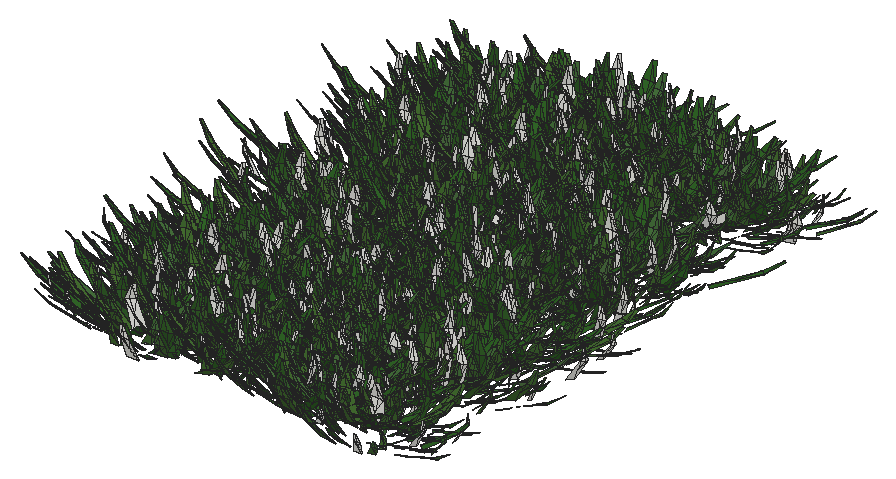
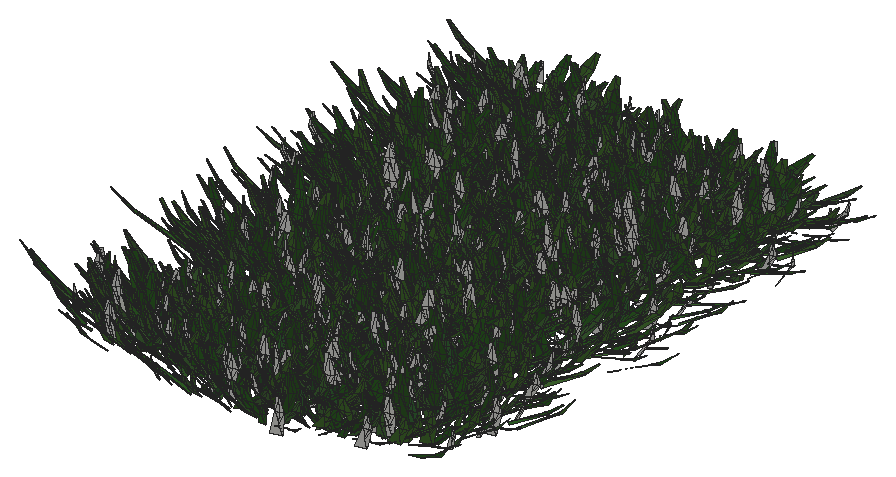
# SketchUp Ruby script. Lengths in inches.
U = 1.inch
M = Sketchup.active_model
def pt(a) = Geom::Point3d.new(a.map { |v| v * U })
def face(e, loops, mat)
  f = e.add_face(loops[0].map { |a| pt(a) })
  loops[1..].each { |l| e.add_face(l.map { |a| pt(a) }).erase! }
  f.material = f.back_material = mat if mat
  f
end
# faces: each face lists its corners as indices into pts; further lists are holes
def faces(e, pts, list, mat = nil) = list.each { |f| face(e, (f[0].is_a?(Array) ? f : [f]).map { |l| l.map { |i| pts[i] } }, mat) }
# xy, xz, yz: faces in a plane at the given z, y or x. An outline is a flat list of corners, or four numbers for a rectangle; further outlines are holes
def ring(l) = l.size == 4 ? [[l[0], l[1]], [l[2], l[1]], [l[2], l[3]], [l[0], l[3]]] : l.each_slice(2).to_a
def flat(e, list, mat, &to3) = list.each { |f| face(e, (f[0].is_a?(Array) ? f : [f]).map { |l| ring(l).map { |u, v| to3.(u, v) } }, mat) }
def xy(e, z, list, mat = nil) = flat(e, list, mat) { |x, y| [x, y, z] }
def xz(e, y, list, mat = nil) = flat(e, list, mat) { |x, z| [x, y, z] }
def yz(e, x, list, mat = nil) = flat(e, list, mat) { |y, z| [x, y, z] }
def lines(e, pts, list) = list.each { |a, b| e.add_line(pt(pts[a]), pt(pts[b])) }
# prism: a flat outline (further loops are holes) pulled along v
def prism(e, loops, v, mat = nil)
  f = face(e, loops, mat); d = Geom::Vector3d.new(v.map { |x| x * U })
  f.pushpull(f.normal.samedirection?(d) ? d.length : -d.length)
end
def box(e, o, s, mat = nil) = prism(e, [[o, [o[0] + s[0], o[1], o[2]], [o[0] + s[0], o[1] + s[1], o[2]], [o[0], o[1] + s[1], o[2]]]], [0, 0, s[2]], mat)
def at(x, y, z, deg = 0) = Geom::Transformation.translation(pt([x, y, z])) * Geom::Transformation.rotation(ORIGIN, Z_AXIS, deg.degrees)
def axes(o, x, y, z) = Geom::Transformation.new([*x, 0, *y, 0, *z, 0, *pt(o).to_a, 1])
def part(name) = M.definitions.add(name)
# library, detail: a bought-in or finely detailed component or shape, given as its bounding box
def library(name, o, s) = part(name).tap { |d| box(d.entities, o, s) }
def detail(e, o, s) = box(e.add_group.entities, o, s)
def put(e, d, t, mat = nil) = e.add_instance(d, t).tap { |i| i.material = mat if mat }
def group(e, t, mat = nil) = e.add_group.tap { |g| g.transformation = t; g.material = mat if mat }.entities
root = M.entities
M.materials.add("Material82").color = [68, 110, 58]
M.materials.add("Material83").color = [48, 90, 38]
M.materials.add("Material84").color = [68, 110, 48]
M.materials.add("Material85").color = [48, 90, 48]
M.materials.add("Material86").color = [58, 110, 58]
M.materials.add("Material87").color = [58, 90, 38]
M.materials.add("Material88").color = [68, 100, 58]
M.materials.add("Material89").color = [48, 100, 38]
c1 = part("grass00")
p = [[-0.6875,0.15,0],[-0.56,0.08,5.52],[-0.04,0.03,2.76],[0.48,-0.02,0],[0.35,-0.02,5.52],[-0.1,-0.14,5.52],
  [-0.12,0.65,8.37],[-0.42,0.65,8.37]]
faces(c1.entities,p,[[0,1,2,3],[3,2,4],[1,5,2],[5,4,2],[1,6,5],[4,5,6],[7,6,1]])
c2 = part("Group16\#1")
put(c2.entities,c1,axes([1.44,-0.61,-0.01],[0.05352,0.12609,0],[-0.10704,0.04543,0.07239],[0.06664,-0.02828,0.11628]),"Material85")
put(c2.entities,c1,axes([0.76,-0.15,-0.01],[0.04676,0.24062,0],[-0.23162,0.04501,0.06642],[0.0652,-0.01267,0.23595]),"Material82")
put(c2.entities,c1,axes([0.79,0.01,-0.01],[-0.00606,0.34651,0],[-0.34381,-0.00602,0.0432],[0.04319,0.00076,0.34386]))
put(c2.entities,c1,axes([1,0.23,-0.01],[-0.07192,0.31144,0],[-0.28722,-0.06632,0.1236],[0.12043,0.02781,0.29478]),"Material84")
put(c2.entities,c1,axes([1.66,0.77,-0.01],[-0.13828,0.29651,0],[-0.21551,-0.1005,0.22471],[0.20365,0.09498,0.23779]),"Material89")
put(c2.entities,c1,axes([0.6875,0.52,-0.01],[-0.18126,0.24051,0],[-0.22746,-0.17142,0.09788],[0.07817,0.05891,0.28481]),"Material84")
put(c2.entities,c1,axes([0.68,0.78,-0.01],[-0.215,0.18688,0],[-0.12385,-0.14248,0.21334],[0.13995,0.16101,0.18878]),"Material82")
put(c2.entities,c1,axes([0.56,1,-0.01],[-0.13756,0.07624,0],[-0.06159,-0.11112,0.0927],[0.04494,0.08108,0.12705]),"Material84")
put(c2.entities,c1,axes([0.2,0.64,-0.01],[-0.23729,0.07254,0],[-0.05711,-0.18681,0.153],[0.04473,0.14632,0.19535]),"Material89")
put(c2.entities,c1,axes([0.0625,0.72,-0.01],[-0.28874,0.02525,0],[-0.02179,-0.24916,0.14647],[0.01276,0.14591,0.25012]),"Material82")
put(c2.entities,c1,axes([-0.08,0.62,-0.01],[-0.34089,-0.04187,0],[0.03255,-0.26504,0.216],[-0.02633,0.21439,0.26703]),"Material89")
put(c2.entities,c1,axes([-0.34,0.98,-0.01],[-0.14314,-0.0493,0],[0.04397,-0.12769,0.06843],[-0.02228,0.0647,0.13505]),"Material89")
put(c2.entities,c1,axes([-0.87,1.45,-0.01],[-0.23488,-0.14114,0],[0.13761,-0.22901,0.06087],[-0.03135,0.05217,0.26717]))
put(c2.entities,c1,axes([-0.72,0.77,-0.01],[-0.14208,-0.13251,0],[0.07209,-0.0773,0.16301],[-0.11118,0.11922,0.1057]),"Material89")
put(c2.entities,c1,axes([-0.62,0.43,-0.01],[-0.14845,-0.21203,0],[0.18654,-0.13061,0.12304],[-0.10079,0.07057,0.22772]),"Material82")
put(c2.entities,c1,axes([-0.68,0.29,-0.01],[-0.13639,-0.32136,0],[0.31723,-0.13464,0.05579],[-0.05136,0.0218,0.34462]),"Material83")
put(c2.entities,c1,axes([-0.64,0.125,-0.01],[-0.0458,-0.23569,0],[0.22124,-0.043,0.08276],[-0.08124,0.01579,0.22538]),"Material86")
put(c2.entities,c1,axes([-1.6,-0.03,-0.01],[0.00576,-0.32897,0],[0.27526,0.00482,0.18018],[-0.18015,-0.00315,0.2753]),"Material84")
put(c2.entities,c1,axes([-1.36,-0.31,-0.01],[0.05718,-0.24765,0],[0.18172,0.04196,0.17267],[-0.16825,-0.03885,0.1865]),"Material89")
put(c2.entities,c1,axes([-1.54,-0.72,-0.01],[0.06537,-0.14017,0],[0.13555,0.06321,0.03939],[-0.0357,-0.01665,0.14956]))
put(c2.entities,c1,axes([-1.19,-0.9,-0.01],[0.09597,-0.12735,0],[0.11214,0.08451,0.07557],[-0.06035,-0.04548,0.14042]),"Material88")
put(c2.entities,c1,axes([-0.47,-0.54,-0.01],[0.11588,-0.10072,0],[0.0618,0.0711,0.12124],[-0.07953,-0.0915,0.0942]))
put(c2.entities,c1,axes([-0.47,-0.84,-0.01],[0.11927,-0.0661,0],[0.06603,0.11913,0.00646],[-0.00313,-0.00565,0.13621]),"Material84")
put(c2.entities,c1,axes([-0.38,-1.24,-0.01],[0.28037,-0.08571,0],[0.0618,0.20215,0.20315],[-0.05939,-0.19428,0.21139]),"Material88")
put(c2.entities,c1,axes([-0.06,-0.66,-0.01],[0.22719,-0.01987,0],[0.01247,0.14255,0.17758],[-0.01547,-0.17691,0.1431]),"Material87")
put(c2.entities,c1,axes([0.11,-0.89,-0.01],[0.14882,0.01828,0],[-0.01058,0.08611,0.12229],[0.01491,-0.12138,0.08676]),"Material85")
put(c2.entities,c1,axes([0.25,-0.72,-0.01],[0.20481,0.07053,0],[-0.06206,0.18022,0.10291],[0.03351,-0.0973,0.1906]),"Material85")
put(c2.entities,c1,axes([0.85,-1.42,-0.01],[0.16481,0.09904,0],[-0.09472,0.15762,0.05616],[0.02893,-0.04814,0.18389]),"Material84")
put(c2.entities,c1,axes([1.01,-1.09,-0.01],[0.21858,0.20385,0],[-0.17495,0.1876,0.15339],[0.10462,-0.11218,0.25652]),"Material89")
put(c2.entities,c1,axes([1.01,-0.71,-0.01],[0.08733,0.12473,0],[-0.06445,0.04512,0.13037],[0.1068,-0.07477,0.07867]),"Material85")
c3 = part("Group15\#1")
put(c3.entities,c2,at(0,0,0))
c4 = part("3darcstudiotree_grass00\#1")
put(c4.entities,c3,at(0,0,0))
put(root,c4,axes([716.16,953.26,-29.74],[1.08587,1.67228,0],[-4.264,0.43062,-0.00469],[-0.02209,0.00223,1.60422]))
put(root,c4,axes([717.65,973.1875,-29.74],[-3.39635,0.60304,0],[-1.8174,-1.59194,-0.05685],[-0.1325,-0.11606,1.88376]))
put(root,c4,axes([716.99,943.77,-29.74],[-0.8053,1.43922,0],[-4.1788,-0.36366,-0.05256],[-0.20936,-0.01822,1.30827]))
put(root,c4,axes([717.81,990.89,-29.74],[1.7154,-1.15643,0],[3.09768,0.71465,-0.02347],[0.14538,0.03354,1.9305]))
put(root,c4,axes([718.48,971.14,-29.74],[-0.55616,-1.38612,0],[4.6364,-0.28933,-0.05346],[0.22148,-0.01382,1.47567]))
put(root,c4,axes([717.84,949.59,-29.74],[2.313,-1.43442,0],[2.99954,0.75225,-0.04064],[0.1888,0.04735,1.46692]))
put(root,c4,axes([717.92,988.37,-29.74],[2.50193,-0.87133,0],[2.32937,1.04026,-0.01409],[0.05813,0.02596,1.64399]))
put(root,c4,axes([718.15,958.98,-29.74],[2.27709,-1.12887,0],[2.96357,0.92974,-0.01848],[0.07518,0.02359,1.47553]))
put(root,c4,axes([717.08,986.68,-29.74],[4.07348,0.57799,0],[-1.18057,1.29405,-0.01256],[-0.02962,0.03247,1.82155]))
put(root,c4,axes([717.24,969.1,-29.74],[2.25028,1.20461,0],[-3.26486,0.94856,-0.0323],[-0.12798,0.03718,1.496]))
put(root,c4,axes([717.87,980.93,-29.74],[-1.39977,1.36626,0],[-3.55438,-0.56636,-0.02451],[-0.1313,-0.02092,1.66036]))
put(root,c4,axes([717.35,950.59,-29.74],[3.43029,0.99275,0],[-1.97308,1.06035,-0.01519],[-0.04853,0.02608,1.34969]))
put(root,c4,axes([718.3125,946.78,-29.74],[-1.21632,1.56365,0],[-3.36368,-0.40694,-0.03727],[-0.21338,-0.02582,1.57911]))
put(root,c4,axes([717.68,963.77,-29.74],[4.01997,0.45296,0],[-1.05214,1.45226,-0.01128],[-0.01738,0.02399,1.61003]))
put(root,c4,axes([718.01,966.45,-29.74],[4.2861,-0.44175,0],[0.90749,1.36943,-0.02428],[0.0455,0.06867,1.99391]))
put(root,c4,axes([718.3125,983.88,-29.74],[3.51248,0.23364,0],[-0.65189,1.52422,-0.03005],[-0.02625,0.06139,1.54341]))
put(root,c4,axes([718.82,942.05,-29.74],[3.31562,-0.63662,0],[1.81859,1.47309,-0.02466],[0.05194,0.04207,1.49812]))
put(root,c4,axes([719.12,977.47,-29.74],[-0.84571,1.33613,0],[-3.59715,-0.35412,-0.00012],[-0.00056,-0.00006,1.39497]))
put(root,c4,axes([719.45,992.93,-29.74],[-1.51727,1.49458,0],[-3.30202,-0.52136,-0.01826],[-0.09361,-0.01478,1.47196]))
put(root,c4,axes([719.8125,955.89,-29.74],[3.22727,-0.96219,0],[2.40393,1.25403,-0.04167],[0.15655,0.08166,1.86151]))
put(root,c4,axes([721.28,953.09,-29.74],[-3.43052,-0.93956,0],[2.00829,-1.14045,-0.00375],[0.01479,-0.0084,1.82358]))
put(root,c4,axes([721.33,946.7,-29.74],[-2.79747,-0.82267,0],[2.4,-1.26929,-0.00029],[0.00098,-0.00052,1.69542]))
put(root,c4,axes([719.71,980.14,-29.74],[3.76479,0.94059,0],[-2.16386,1.34705,-0.03414],[-0.08584,0.05343,1.42377]))
put(root,c4,axes([721.42,960.45,-29.74],[-3.74102,0.70585,0],[-1.92999,-1.5909,-0.05113],[-0.08819,-0.0727,1.33965]))
put(root,c4,axes([721.69,982.32,-29.74],[2.94171,-1.11183,0],[3.18535,1.31078,-0.03986],[0.13301,0.05473,1.66404]))
put(root,c4,axes([722.18,941.6875,-29.74],[-3.65106,0.9561,0],[-2.55118,-1.5152,-0.05111],[-0.12576,-0.07469,1.53759]))
put(root,c4,axes([722.15,968.48,-29.74],[-2.1448,1.18286,0],[-3.37437,-0.95161,-0.05929],[-0.21963,-0.06194,1.41608]))
put(root,c4,axes([721.3125,951.12,-29.74],[2.61816,1.29298,0],[-2.60516,0.82044,-0.01421],[-0.06264,0.01973,1.40932]))
put(root,c4,axes([723.09,983.85,-29.74],[-0.23596,-1.70659,0],[3.32039,-0.0714,-0.01049],[0.06174,-0.00133,1.4693]))
put(root,c4,axes([724,985.85,-29.74],[-2.68837,-0.8629,0],[2.90522,-1.40773,-0.04334],[0.1065,-0.05161,1.34295]))
put(root,c4,axes([723.33,980.02,-29.74],[2.30193,-1.12166,0],[3.41965,1.0915,-0.0352],[0.15447,0.0493,1.86157]))
put(root,c4,axes([724.3,977.03,-29.74],[-3.8851,-1.03716,0],[2.44189,-1.42264,-0.04034],[0.11257,-0.06558,1.62559]))
put(root,c4,axes([722.23,957.93,-29.74],[4.25337,0.6683,0],[-1.56461,1.54873,-0.01606],[-0.02903,0.02874,1.54782]))
put(root,c4,axes([722.53,975.2,-29.74],[0.91536,1.26151,0],[-4.37209,0.4934,-0.02742],[-0.14974,0.0169,1.93645]))
put(root,c4,axes([722.78,966.12,-29.74],[-0.09975,1.34747,0],[-4.08432,-0.04703,-0.00454],[-0.02466,-0.00028,1.66362]))
put(root,c4,axes([724.77,964.17,-29.74],[-1.28823,-1.73919,0],[3.44626,-0.39701,-0.03009],[0.18497,-0.02131,1.72353]))
put(root,c4,axes([723.67,995.19,-29.74],[3.82297,0.44431,0],[-0.93883,1.25636,-0.026],[-0.04711,0.06304,1.59572]))
put(root,c4,axes([725.2,991.98,-29.74],[1.61408,-1.6002,0],[4.35972,0.68394,-0.04298],[0.19186,0.0301,1.68954]))
put(root,c4,axes([723.86,989.56,-29.74],[4.08766,0.51132,0],[-1.24704,1.55051,-0.00141],[-0.00269,0.00335,1.95289]))
put(root,c4,axes([724.34,944.97,-29.74],[0.40934,1.39565,0],[-3.638,0.16595,-0.04522],[-0.26335,0.01201,1.60941]))
put(root,c4,axes([724.75,949.33,-29.74],[-2.97215,1.15542,0],[-3.15373,-1.26173,-0.01243],[-0.04576,-0.01831,1.76595]))
put(root,c4,axes([724.76,987.72,-29.74],[4.03922,-0.03156,0],[0.07296,1.45219,-0.01855],[0.00258,0.0513,1.93628]))
put(root,c4,axes([724.84,955.45,-29.74],[1.39622,1.62786,0],[-3.6301,0.48424,-0.04556],[-0.23124,0.03085,1.53888]))
put(root,c4,axes([725.35,961.14,-29.74],[4.28281,-0.63976,0],[1.42181,1.48036,-0.01068],[0.01649,0.01717,1.31138]))
put(root,c4,axes([725.31,973.6,-29.74],[3.35774,0.54146,0],[-1.57719,1.52117,-0.03911],[-0.07127,0.06874,1.50402]))
put(root,c4,axes([727.24,964.76,-29.74],[-1.97401,-1.44609,0],[3.51216,-0.74566,-0.02018],[0.11603,-0.02463,1.95264]))
put(root,c4,axes([727.18,979.34,-29.74],[-2.39621,-0.97294,0],[2.61152,-1.00033,-0.02073],[0.08443,-0.03234,1.5494]))
put(root,c4,axes([725.23,970.62,-29.74],[2.01516,1.65729,0],[-3.55056,0.67146,-0.00104],[-0.005,0.00095,1.58037]))
put(root,c4,axes([727.72,976.84,-29.74],[-3.41262,-0.98405,0],[2.00346,-1.0806,-0.03203],[0.14502,-0.07822,1.95145]))
put(root,c4,axes([726.91,942.67,-29.74],[3.35024,-0.43777,0],[1.10858,1.31952,-0.03222],[0.06859,0.08164,1.78787]))
put(root,c4,axes([727.55,994.33,-29.74],[2.23301,-1.20393,0],[2.80312,0.80861,-0.02877],[0.133,0.03837,1.49076]))
put(root,c4,axes([729.01,973.25,-29.74],[-1.89614,-1.52378,0],[3.69892,-0.71587,-0.01008],[0.04587,-0.00888,1.566]))
put(root,c4,axes([727.42,946.05,-29.74],[0.10079,1.33733,0],[-4.05045,0.04748,-0.05613],[-0.28184,0.0033,1.5259]))
put(root,c4,axes([728.13,967.75,-29.74],[3.01451,-0.88182,0],[2.30556,1.22582,-0.02804],[0.08966,0.04767,1.55696]))
put(root,c4,axes([727.36,945.2,-29.74],[2.52987,0.96809,0],[-2.35442,0.95693,-0.00683],[-0.03278,0.01332,1.74693]))
put(root,c4,axes([728.88,990.53,-29.74],[-4.40755,0.3662,0],[-0.80873,-1.51388,-0.00142],[-0.00162,-0.00303,1.63114]))
put(root,c4,axes([729.15,970.07,-29.74],[-3.86461,-0.59074,0],[1.45311,-1.4785,-0.05586],[0.12869,-0.13094,1.92103]))
put(root,c4,axes([729.28,954.54,-29.74],[0.04452,-1.40138,0],[3.5701,0.01764,-0.00992],[0.04898,0.00024,1.32167]))
put(root,c4,axes([729,992.66,-29.74],[-3.74567,1.07998,0],[-2.52019,-1.35944,-0.03994],[-0.14532,-0.07839,1.97331]))
put(root,c4,axes([727.96,985.13,-29.74],[4.59378,0.22046,0],[-0.54654,1.77125,-0.0359],[-0.02405,0.07793,1.88046]))
put(root,c4,axes([729.3,980.81,-29.74],[1.47145,-1.32607,0],[3.01918,0.52105,-0.00213],[0.01031,0.00178,1.30651]))
put(root,c4,axes([730.42,948.32,-29.74],[-2.64283,-1.13535,0],[3.48014,-1.25993,-0.02326],[0.08818,-0.03192,1.82249]))
put(root,c4,axes([729.875,951.53,-29.74],[1.26532,-1.44178,0],[3.12553,0.42661,-0.00044],[0.00223,0.0003,1.32507]))
put(root,c4,axes([730.39,961.61,-29.74],[-4.13794,-0.2249,0],[0.58111,-1.66288,-0.00876],[0.00496,-0.01418,1.32289]))
put(root,c4,axes([729.44,983.75,-29.74],[-2.89048,1.44179,0],[-2.90546,-0.90593,-0.0043],[-0.02277,-0.0071,1.8735]))
put(root,c4,axes([728.53,975.54,-29.74],[2.24895,1.38406,0],[-3.92977,0.99312,-0.02786],[-0.13256,0.0335,1.9768]))
put(root,c4,axes([729.49,952.74,-29.74],[3.40614,0.32781,0],[-0.81542,1.31776,-0.01459],[-0.02356,0.03807,1.75568]))
put(root,c4,axes([729.57,996.99,-29.74],[4.11101,0.00408,0],[-0.01055,1.6533,-0.01268],[-0.00019,0.02913,1.83013]))
put(root,c4,axes([729.71,988.6875,-29.74],[4.61322,-0.12203,0],[0.30512,1.79396,-0.00473],[0.00139,0.00815,1.49489]))
put(root,c4,axes([729.63,957.56,-29.74],[3.60093,0.62069,0],[-1.54425,1.39338,-0.01451],[-0.03218,0.02903,1.59989]))
put(root,c4,axes([730.73,960.13,-29.74],[-0.93158,1.57452,0],[-3.64716,-0.33561,-0.02125],[-0.09909,-0.00912,1.34411]))
put(root,c4,axes([730.61,965.66,-29.74],[1.53583,1.49996,0],[-3.93703,0.62697,-0.05886],[-0.22971,0.03658,1.33951]))
put(root,c4,axes([732.86,959.57,-29.74],[-2.29669,-1.11112,0],[2.95834,-0.95105,-0.00371],[0.01505,-0.00484,1.4993]))
put(root,c4,axes([732.79,994.95,-29.74],[-2.49297,-0.95003,0],[2.84759,-1.16217,-0.03177],[0.13042,-0.05323,1.8145]))
put(root,c4,axes([732.6,965.81,-29.74],[-2.8718,1.45727,0],[-2.81901,-0.86401,-0.03149],[-0.12433,-0.03811,1.33797]))
put(root,c4,axes([732.55,957.45,-29.74],[-2.73949,1.39402,0],[-3.69271,-1.12865,-0.03455],[-0.12332,-0.03769,1.58129]))
put(root,c4,axes([733.99,985.67,-29.74],[-2.79426,-0.70511,0],[1.77672,-1.09506,-0.02395],[0.07288,-0.04492,1.39534]))
put(root,c4,axes([732.8,948.12,-29.74],[4.32757,-0.42653,0],[1.12297,1.77206,-0.03338],[0.0321,0.05066,1.37691]))
put(root,c4,axes([733.07,974.3,-29.74],[3.39282,-0.2362,0],[0.75884,1.6953,-0.03701],[0.03902,0.08718,1.98432]))
put(root,c4,axes([733.02,983.04,-29.74],[1.01985,1.24994,0],[-3.27441,0.41552,-0.0339],[-0.22651,0.02874,1.80984]))
put(root,c4,axes([733.47,955.09,-29.74],[3.17214,0.39156,0],[-1.05658,1.33127,-0.01935],[-0.04192,0.05282,1.92273]))
put(root,c4,axes([733.78,972.06,-29.74],[3.44047,-0.2055,0],[0.68194,1.77564,-0.05863],[0.04271,0.1112,1.66018]))
put(root,c4,axes([734.59,992.99,-29.74],[-2.53173,1.21264,0],[-2.8931,-0.93942,-0.04557],[-0.23211,-0.07537,1.85346]))
put(root,c4,axes([735.34,946.88,-29.74],[-3.83423,-0.51133,0],[1.38691,-1.61748,-0.06149],[0.1095,-0.1277,1.80385]))
put(root,c4,axes([735.45,971.34,-29.74],[-2.06404,-1.37727,0],[3.69374,-0.86095,-0.04139],[0.20463,-0.0477,1.84708]))
put(root,c4,axes([733.65,981.04,-29.74],[2.13019,1.09948,0],[-3.08878,0.93074,-0.0123],[-0.05365,0.01617,1.59876]))
put(root,c4,axes([735.73,987.38,-29.74],[-4.29389,-0.13256,0],[0.34176,-1.72178,-0.05117],[0.01874,-0.09441,1.54048]))
put(root,c4,axes([734.36,942.03,-29.74],[4.09444,0.12503,0],[-0.31641,1.61154,-0.0417],[-0.02006,0.10219,1.91485]))
put(root,c4,axes([735.71,967.74,-29.74],[-3.97452,0.57658,0],[-1.26948,-1.361,-0.04924],[-0.12234,-0.13116,1.98345]))
put(root,c4,axes([734.44,979.83,-29.74],[4.64305,-0.03413,0],[0.08366,1.7702,-0.03615],[0.00311,0.0658,1.55355]))
put(root,c4,axes([734.28,944.35,-29.74],[3.61655,0.77067,0],[-2.16585,1.58076,-0.05913],[-0.11484,0.08382,1.39517]))
put(root,c4,axes([735.71,950.95,-29.74],[-3.45507,0.18922,0],[-0.60525,-1.7188,-0.02154],[-0.01288,-0.03658,1.4342]))
put(root,c4,axes([736.1,996.36,-29.74],[-3.18702,-0.48311,0],[1.45771,-1.49562,-0.04802],[0.08757,-0.08985,1.54794]))
put(root,c4,axes([735.09,952.61,-29.74],[1.33968,1.52005,0],[-3.16755,0.43419,-0.01128],[-0.07711,0.01057,1.81963]))
put(root,c4,axes([735.66,962.625,-29.74],[-0.83712,1.35251,0],[-3.5635,-0.34303,-0.03757],[-0.17469,-0.01682,1.3158]))
put(root,c4,axes([736.42,964.89,-29.74],[3.08356,-0.59749,0],[1.85245,1.48689,-0.05746],[0.15906,0.12767,1.97658]))
put(root,c4,axes([736.31,977.9,-29.74],[1.55645,1.18195,0],[-3.2541,0.66647,-0.04821],[-0.21297,0.04362,1.36797]))
put(root,c4,axes([736.44,990.47,-29.74],[0.845,1.27042,0],[-4.02841,0.41673,-0.05161],[-0.24313,0.02515,1.52021]))
put(root,c4,axes([738.64,970.42,-29.74],[-3.70591,-0.99796,0],[1.87776,-1.08451,-0.01838],[0.07513,-0.04339,1.80866]))
put(root,c4,axes([738.66,986.51,-29.74],[0.0983,-1.39772,0],[3.56781,0.03903,-0.00183],[0.01012,0.00011,1.48199]))
put(root,c4,axes([738.35,951.6875,-29.74],[2.17735,-1.14497,0],[3.55677,1.05197,-0.03529],[0.11494,0.03399,1.35654]))
put(root,c4,axes([739.28,964.24,-29.74],[-4.087,-0.33484,0],[0.93219,-1.7696,-0.02537],[0.02744,-0.05209,1.82613]))
put(root,c4,axes([738.95,975.18,-29.74],[-3.8828,0.51827,0],[-1.09306,-1.27365,-0.02484],[-0.06133,-0.07146,1.96802]))
put(root,c4,axes([739.23,955.43,-29.74],[-4.01589,0.275,0],[-0.74615,-1.69466,-0.05401],[-0.03733,-0.08478,1.3206]))
put(root,c4,axes([738.67,960.24,-29.74],[-1.92395,1.11114,0],[-2.73961,-0.73778,-0.01899],[-0.11099,-0.02989,1.75992]))
put(root,c4,axes([738,941.76,-29.74],[-0.14266,1.36173,0],[-4.10184,-0.06683,-0.00296],[-0.01424,-0.00023,1.47961]))
put(root,c4,axes([738.27,965.58,-29.74],[-0.37072,1.84099,0],[-4.27519,-0.13389,-0.01448],[-0.06545,-0.00205,1.45727]))
put(root,c4,axes([738.48,994.4,-29.74],[4.18586,0.29447,0],[-0.62505,1.38186,-0.04495],[-0.05854,0.12943,1.97854]))
put(root,c4,axes([740.56,967.85,-29.74],[-0.69027,-1.34957,0],[4.18043,-0.33255,-0.04603],[0.23408,-0.01862,1.65834]))
put(root,c4,axes([739.17,943.8,-29.74],[3.68364,0.44666,0],[-1.28613,1.64968,-0.02064],[-0.02718,0.03487,1.46981]))
put(root,c4,axes([740.51,981.01,-29.74],[-3.79382,0.9598,0],[-2.14839,-1.32076,-0.01729],[-0.051,-0.03135,1.62898]))
put(root,c4,axes([741.16,952.49,-29.74],[-3.50392,-0.27669,0],[0.88512,-1.7433,-0.02406],[0.02146,-0.04227,1.53532]))
put(root,c4,axes([741.43,988.08,-29.74],[-4.49069,-0.28234,0],[0.61208,-1.5141,-0.05098],[0.04605,-0.11392,1.67187]))
put(root,c4,axes([739.98,977.58,-29.74],[4.2001,-0.13479,0],[0.33266,1.61217,-0.01977],[0.00834,0.04041,1.59866]))
put(root,c4,axes([741.25,979.17,-29.74],[-4.51566,0.3438,0],[-0.75132,-1.53478,-0.00152],[-0.00137,-0.0028,1.41339]))
put(root,c4,axes([740.19,972,-29.74],[-1.23007,1.60855,0],[-3.72331,-0.44283,-0.01363],[-0.06328,-0.00753,1.41312]))
put(root,c4,axes([740.875,946.86,-29.74],[-2.10873,0.99525,0],[-2.92476,-0.96381,-0.03387],[-0.14037,-0.04626,1.54303]))
put(root,c4,axes([740.72,949.03,-29.74],[3.33633,-0.58263,0],[1.85643,1.65335,-0.04981],[0.10311,0.09183,1.75709]))
put(root,c4,axes([740.4,983.75,-29.74],[2.36553,1.18037,0],[-3.06807,0.95629,-0.02315],[-0.10187,0.03175,1.64391]))
put(root,c4,axes([740.28,992.54,-29.74],[2.70315,0.92974,0],[-3.09727,1.40055,-0.01764],[-0.05733,0.02592,1.74631]))
put(root,c4,axes([741.57,961.79,-29.74],[2.84805,-1.35819,0],[2.78081,0.90692,-0.04304],[0.21584,0.07039,1.76026]))
put(root,c4,axes([741.02,956.85,-29.74],[0.25957,1.50579,0],[-3.94932,0.10588,-0.02807],[-0.1244,0.00334,1.3177]))
put(root,c4,axes([743.625,942.74,-29.74],[-2.56709,-0.87628,0],[2.75862,-1.25691,-0.00422],[0.01164,-0.0053,1.33295]))
put(root,c4,axes([741.91,990.16,-29.74],[3.46346,0.58344,0],[-1.61207,1.48838,-0.00364],[-0.00911,0.00841,1.96053]))
put(root,c4,axes([744.75,988.43,-29.74],[-2.62594,-1.45094,0],[3.42478,-0.964,-0.01802],[0.06257,-0.01761,1.345]))
put(root,c4,axes([744.26,979.68,-29.74],[-3.57945,0.04189,0],[-0.11544,-1.5341,-0.02538],[-0.0045,-0.05977,1.74242]))
put(root,c4,axes([743.52,957.48,-29.74],[-2.10864,1.34219,0],[-3.56504,-0.87109,-0.01218],[-0.05259,-0.01285,1.59607]))
put(root,c4,axes([744.23,951.41,-29.74],[3.4734,-0.75241,0],[2.06047,1.47936,-0.02691],[0.07219,0.05183,1.78778]))
put(root,c4,axes([745.51,944.38,-29.74],[-1.56362,-1.21345,0],[3.6466,-0.73082,-0.00876],[0.03709,-0.00743,1.45672]))
put(root,c4,axes([745.74,959.59,-29.74],[-3.17921,-1.35137,0],[3.1644,-1.15784,-0.01209],[0.04457,-0.01631,1.62724]))
put(root,c4,axes([745.8,963.76,-29.74],[-2.5712,-1.27561,0],[3.33499,-1.0455,-0.01168],[0.0385,-0.01207,1.34439]))
put(root,c4,axes([744.11,974.79,-29.74],[-0.16089,1.57179,0],[-4.27524,-0.06806,-0.04298],[-0.25282,-0.00402,1.88799]))
put(root,c4,axes([745.85,968.13,-29.74],[-3.47552,-0.34069,0],[1.08655,-1.72393,-0.01735],[0.02109,-0.03347,1.70162]))
put(root,c4,axes([745.76,971.25,-29.74],[-3.29266,-0.34854,0],[0.95777,-1.40726,-0.03217],[0.05606,-0.08237,1.86146]))
put(root,c4,axes([744,949.47,-29.74],[2.09092,1.38555,0],[-3.43654,0.80658,-0.00188],[-0.01015,0.00238,1.87843]))
put(root,c4,axes([744.4,972.92,-29.74],[1.95292,1.06951,0],[-2.86765,0.8144,-0.02117],[-0.10996,0.03123,1.69559]))
put(root,c4,axes([745.07,961.49,-29.74],[-1.97289,1.32597,0],[-3.97358,-0.91953,-0.01374],[-0.05147,-0.01191,1.50009]))
put(root,c4,axes([744.71,940.58,-29.74],[0.75696,1.65896,0],[-4.64105,0.32936,-0.03105],[-0.12997,0.00922,1.50318]))
put(root,c4,axes([744.9,977.4,-29.74],[4.5376,0.13529,0],[-0.33368,1.74059,-0.04634],[-0.02094,0.10925,1.98901]))
put(root,c4,axes([745.03,986.54,-29.74],[1.35175,1.46561,0],[-4.38115,0.62846,-0.0524],[-0.19286,0.02766,1.36852]))
put(root,c4,axes([746.93,990.7,-29.74],[-4.23196,-0.66829,0],[1.43136,-1.40974,-0.04264],[0.09281,-0.09141,1.69007]))
put(root,c4,axes([745.95,993.125,-29.74],[2.88826,-0.72218,0],[1.92215,1.1956,-0.03299],[0.1167,0.07259,1.77748]))
put(root,c4,axes([746.52,953.89,-29.74],[-2.97303,0.61552,0],[-2.04085,-1.53313,-0.02543],[-0.06857,-0.05151,1.9093]))
put(root,c4,axes([745.81,994.58,-29.74],[1.93247,1.08024,0],[-2.71059,0.75417,-0.03223],[-0.14585,0.04058,1.37708]))
